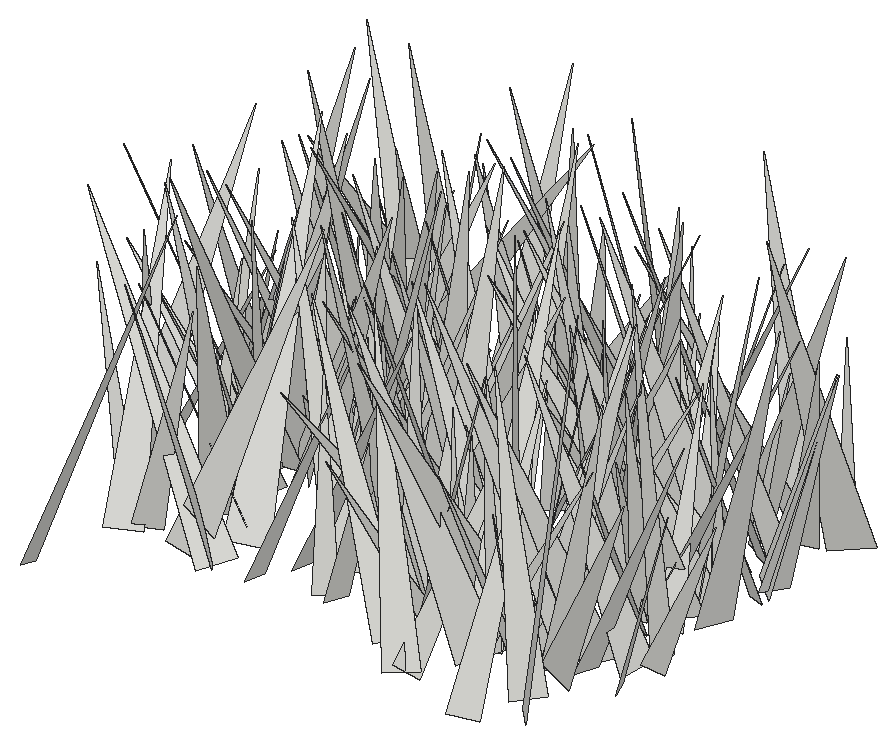
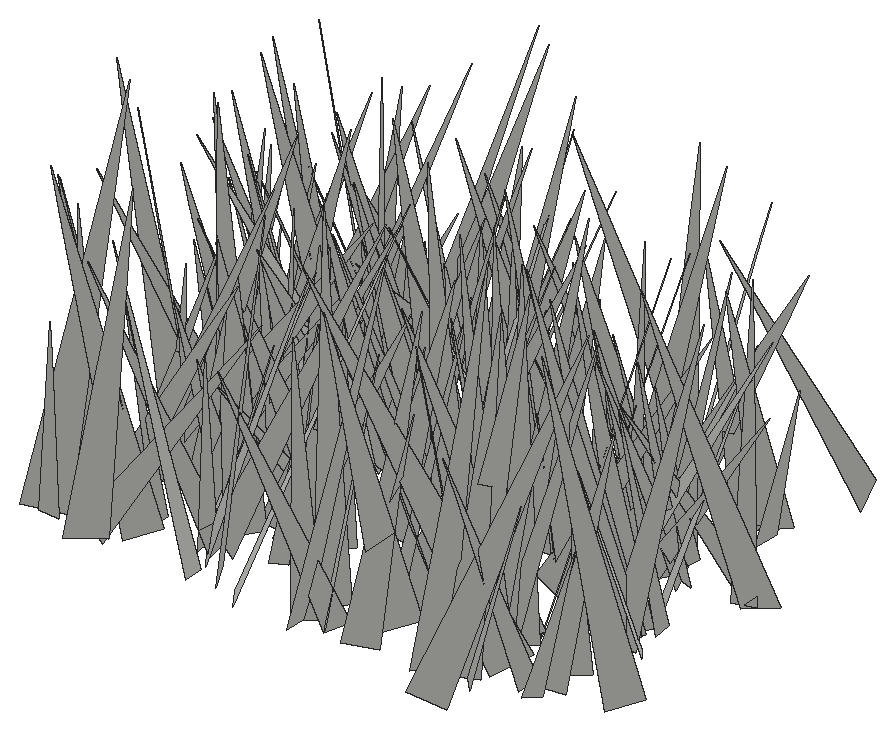
# SketchUp Ruby script. Lengths in inches.
U = 1.inch
M = Sketchup.active_model
def pt(a) = Geom::Point3d.new(a.map { |v| v * U })
def face(e, loops, mat)
  f = e.add_face(loops[0].map { |a| pt(a) })
  loops[1..].each { |l| e.add_face(l.map { |a| pt(a) }).erase! }
  f.material = f.back_material = mat if mat
  f
end
# faces: each face lists its corners as indices into pts; further lists are holes
def faces(e, pts, list, mat = nil) = list.each { |f| face(e, (f[0].is_a?(Array) ? f : [f]).map { |l| l.map { |i| pts[i] } }, mat) }
# xy, xz, yz: faces in a plane at the given z, y or x. An outline is a flat list of corners, or four numbers for a rectangle; further outlines are holes
def ring(l) = l.size == 4 ? [[l[0], l[1]], [l[2], l[1]], [l[2], l[3]], [l[0], l[3]]] : l.each_slice(2).to_a
def flat(e, list, mat, &to3) = list.each { |f| face(e, (f[0].is_a?(Array) ? f : [f]).map { |l| ring(l).map { |u, v| to3.(u, v) } }, mat) }
def xy(e, z, list, mat = nil) = flat(e, list, mat) { |x, y| [x, y, z] }
def xz(e, y, list, mat = nil) = flat(e, list, mat) { |x, z| [x, y, z] }
def yz(e, x, list, mat = nil) = flat(e, list, mat) { |y, z| [x, y, z] }
def lines(e, pts, list) = list.each { |a, b| e.add_line(pt(pts[a]), pt(pts[b])) }
# prism: a flat outline (further loops are holes) pulled along v
def prism(e, loops, v, mat = nil)
  f = face(e, loops, mat); d = Geom::Vector3d.new(v.map { |x| x * U })
  f.pushpull(f.normal.samedirection?(d) ? d.length : -d.length)
end
def box(e, o, s, mat = nil) = prism(e, [[o, [o[0] + s[0], o[1], o[2]], [o[0] + s[0], o[1] + s[1], o[2]], [o[0], o[1] + s[1], o[2]]]], [0, 0, s[2]], mat)
def at(x, y, z, deg = 0) = Geom::Transformation.translation(pt([x, y, z])) * Geom::Transformation.rotation(ORIGIN, Z_AXIS, deg.degrees)
def axes(o, x, y, z) = Geom::Transformation.new([*x, 0, *y, 0, *z, 0, *pt(o).to_a, 1])
def part(name) = M.definitions.add(name)
# library, detail: a bought-in or finely detailed component or shape, given as its bounding box
def library(name, o, s) = part(name).tap { |d| box(d.entities, o, s) }
def detail(e, o, s) = box(e.add_group.entities, o, s)
def put(e, d, t, mat = nil) = e.add_instance(d, t).tap { |i| i.material = mat if mat }
def group(e, t, mat = nil) = e.add_group.tap { |g| g.transformation = t; g.material = mat if mat }.entities
root = M.entities
c1 = part("fur_instance\#9")
p = [[0.8125,0,1.79],[0.67,-0.02,1.48],[0,-0.11,0],[0,0.11,0]]
faces(c1.entities,p,[[0,1,2,3]])
put(root,c1,axes([528.22,20.27,-21.86],[6.68377,2.4417,1.0502],[1.89436,-6.36953,2.75283],[-1.86446,2.28139,6.56175]))
put(root,c1,axes([533.33,24.67,-21.86],[-4.99483,-3.69291,1.05885],[-3.66459,5.10128,0.50484],[1.15306,0.21561,6.19121]))
put(root,c1,axes([545.3125,25.14,-21.86],[-6.87965,3.10007,2.46286],[3.78941,6.58637,2.29475],[1.14737,-3.16466,7.18848]))
put(root,c1,axes([548.58,25.63,-21.86],[0.60809,-6.43634,0.77652],[-5.71222,-0.16309,3.1214],[3.06594,0.97271,5.66154]))
put(root,c1,axes([543.94,22.4375,-21.86],[-2.77056,6.19265,0.76015],[6.19361,2.62958,1.15202],[-0.75223,-1.15721,6.68563]))
put(root,c1,axes([544.375,28.09,-21.86],[-7.59167,-1.95799,2.55179],[-0.44126,7.11339,4.14535],[3.18601,-3.68034,6.65457]))
put(root,c1,axes([548.18,24.13,-21.86],[-2.17091,-2.72609,1.07786],[-2.90812,2.17161,-0.36485],[0.36901,1.07644,3.46573]))
put(root,c1,axes([541.78,26.45,-21.86],[-4.13984,-2.04423,0.54277],[-1.65039,3.86825,1.98107],[1.32277,-1.57147,4.17043]))
put(root,c1,axes([548.81,23.75,-21.86],[-4.49758,4.50366,1.60112],[4.72062,4.53017,0.51777],[0.74986,-1.50644,6.34374]))
put(root,c1,axes([548.17,24.49,-21.86],[-1.77005,-3.87903,0.89181],[-3.77258,1.32393,-1.7292],[-1.26879,1.475,3.89741]))
put(root,c1,axes([549.52,22.64,-21.86],[5.31201,5.41879,2.20999],[5.24419,-5.73235,1.45032],[-2.59727,-0.49162,7.44831]))
put(root,c1,axes([530,25.04,-21.86],[3.51302,-4.23345,1.0034],[-4.35037,-3.40123,0.88101],[0.05668,1.33409,5.43021]))
put(root,c1,axes([547.81,21.18,-21.86],[-5.23053,3.77379,0.03544],[3.44734,4.80229,-2.57973],[1.53577,2.07308,5.91142]))
put(root,c1,axes([542.18,24.05,-21.86],[-3.49983,5.63032,0.78088],[5.54982,3.18646,1.89866],[-1.22869,-1.64469,6.35172]))
put(root,c1,axes([531.5,27.51,-21.86],[4.72004,-5.82808,0.22381],[-5.80637,-4.72269,-0.52693],[-0.55017,-0.15829,7.48115]))
put(root,c1,axes([532.24,24.45,-21.86],[-0.29437,7.39176,2.68978],[7.28817,1.26884,-2.68928],[2.95898,-2.3899,6.89148]))
put(root,c1,axes([533.66,24.48,-21.86],[-4.54084,5.90887,0.08971],[5.53212,4.21055,2.68494],[-2.07809,-1.7025,6.95162]))
put(root,c1,axes([542.27,25.55,-21.86],[5.73054,2.09287,1.0832],[2.24178,-5.71944,-0.8093],[-0.7265,-1.14039,6.04684]))
put(root,c1,axes([538.19,25.17,-21.86],[-2.40866,3.6867,1.3913],[3.88066,2.50239,0.08743],[0.68406,-1.21467,4.40293]))
put(root,c1,axes([535.37,24.59,-21.86],[5.62442,0.34622,0.61815],[0.22701,-5.5658,1.05184],[-0.67115,1.01884,5.53603]))
put(root,c1,axes([545.3,25.47,-21.86],[3.75203,3.55416,0.24846],[3.4305,-3.50645,-1.64561],[0.96201,-1.35805,4.89916]))
put(root,c1,axes([549.14,27.58,-21.86],[2.35436,-6.19743,2.05043],[-5.78585,-2.99044,-2.39512],[-3.02263,0.89697,6.18179]))
put(root,c1,axes([539.05,29.83,-21.86],[-5.34969,-3.46152,0.37635],[-2.75195,4.62606,3.43064],[2.1332,-2.713,5.36954]))
put(root,c1,axes([548.21,26.17,-21.86],[5.31281,-2.73186,1.51927],[-2.91837,-5.40827,0.48055],[-1.11999,1.13346,5.95467]))
put(root,c1,axes([548.04,27.38,-21.86],[-8.03194,-0.35365,0.82088],[-0.22203,7.97883,1.26494],[0.86581,-1.23463,7.93959]))
put(root,c1,axes([540.31,27.43,-21.86],[-1.48143,-7.59825,2.03928],[-7.84224,1.26126,-0.99758],[-0.62555,2.18232,7.67677]))
put(root,c1,axes([536.26,26.47,-21.86],[6.32443,-0.86949,0.03215],[-0.87008,-6.31952,0.24926],[0.00213,0.25131,6.37905]))
put(root,c1,axes([529.03,25.28,-21.86],[-4.67353,1.04438,0.03845],[1.02272,4.60667,-0.8165],[0.21505,0.78861,4.71868]))
put(root,c1,axes([545.79,25.68,-21.86],[-4.82421,0.67017,1.12309],[0.52178,4.9221,-0.69578],[1.19925,0.5543,4.82058]))
put(root,c1,axes([544.24,25.28,-21.86],[0.68638,4.30492,0.85677],[4.11958,-0.93113,1.37825],[-1.51508,-0.58153,4.13569]))
put(root,c1,axes([544.08,22.53,-21.86],[-5.06896,3.36354,0.19703],[2.56301,4.08037,-3.71862],[2.18706,3.01393,4.81452]))
put(root,c1,axes([550.95,26.39,-21.86],[3.66327,1.41122,0.72087],[1.44956,-3.71776,-0.08822],[-0.64027,-0.34277,3.92471]))
put(root,c1,axes([529.375,24.4,-21.86],[-3.85678,5.81728,0.33644],[5.7739,3.8696,-0.71896],[0.78484,0.11882,6.94252]))
put(root,c1,axes([550.54,27.97,-21.86],[-6.51837,1.52305,1.37348],[1.82295,6.39951,1.5551],[0.93967,-1.84981,6.5108]))
put(root,c1,axes([547.09,25.1875,-21.86],[-7.31055,-2.64435,2.80127],[-3.45475,7.15889,-2.25809],[1.70424,3.16886,7.43894]))
put(root,c1,axes([532.53,27.58,-21.86],[-3.6362,-3.51378,0.23491],[-3.4583,3.49912,-1.19165],[-0.6648,1.01649,4.91412]))
put(root,c1,axes([549.14,26.72,-21.86],[5.55155,-0.72144,0.45458],[-0.77671,-5.51397,0.73462],[-0.35191,0.78896,5.54982]))
put(root,c1,axes([545.98,26.65,-21.86],[-4.87029,1.64927,0.93909],[1.65484,4.95663,-0.12272],[0.92923,-0.18296,5.1405]))
put(root,c1,axes([542.8,27.73,-21.86],[2.98723,-2.64764,1.00912],[-2.72025,-3.09017,-0.05514],[-0.79284,0.62671,3.99131]))
put(root,c1,axes([542.49,28.64,-21.86],[-3.80657,-5.75041,0.9295],[-5.82495,3.76407,-0.56819],[0.03325,1.08891,6.87272]))
put(root,c1,axes([546.9,27.07,-21.86],[3.44666,-5.98968,2.82803],[-6.61551,-2.95389,1.80641],[0.33028,3.33943,6.67028]))
put(root,c1,axes([538.6875,25.21,-21.86],[-7.17026,0.40545,3.85637],[-0.86926,7.73252,-2.42922],[3.77894,2.54801,6.75839]))
put(root,c1,axes([539.45,29.11,-21.86],[4.28198,-1.79299,1.3249],[-1.43721,-4.41332,-1.32759],[-1.70429,-0.78312,4.44833]))
put(root,c1,axes([551.01,28.27,-21.86],[2.19638,-3.75423,0.49776],[-3.62923,-1.92217,1.51658],[1.08198,1.1735,4.07656]))
put(root,c1,axes([539.53,27.79,-21.86],[-3.51582,-2.14374,0.80605],[-2.26912,3.46073,-0.69338],[0.31056,1.01688,4.05904]))
put(root,c1,axes([537.68,26.9,-21.86],[-2.86561,6.0597,1.12131],[6.09085,2.59686,1.53195],[-0.93747,-1.65086,6.5257]))
put(root,c1,axes([526.68,29.48,-21.86],[-0.27546,-6.0552,1.07535],[-6.00995,0.49341,1.23885],[1.30474,0.99438,5.93351]))
put(root,c1,axes([546.91,26.4375,-21.86],[3.10305,4.72146,0.30771],[4.72969,-3.10544,-0.04628],[-0.13026,-0.28259,5.64969]))
put(root,c1,axes([538.18,28.74,-21.86],[-0.76363,-5.08076,1.72351],[-5.30047,0.98391,0.55201],[0.83046,1.60796,5.10809]))
put(root,c1,axes([540.88,26.92,-21.86],[-5.6137,1.8249,1.28834],[1.63706,5.7317,-0.98561],[1.51991,0.56669,5.82001]))
put(root,c1,axes([545.02,25.62,-21.86],[-2.31741,7.72302,0.72504],[7.71845,2.37113,-0.58682],[0.77216,-0.52327,8.04183]))
put(root,c1,axes([548.56,30.52,-21.86],[-1.70648,-4.83175,0.15849],[-4.67215,1.69151,1.26205],[1.24174,-0.27565,4.96639]))
put(root,c1,axes([531.08,31.69,-21.86],[0.62863,-8.27068,0.12443],[-8.26435,-0.63324,-0.33804],[-0.34653,0.09834,8.28764]))
put(root,c1,axes([531.95,30.14,-21.86],[2.79879,-2.29313,0.37979],[-2.08936,-2.74248,-1.16161],[-1.01846,-0.6755,3.42672]))
put(root,c1,axes([535.9375,27.78,-21.86],[3.61402,1.40651,0.81578],[1.29809,-3.69316,0.61679],[-0.97915,0.29527,3.8287]))
put(root,c1,axes([537.5,33.42,-21.86],[-5.2335,-6.40482,0.23356],[-5.52847,4.66397,4.0186],[3.24225,-2.38569,7.22925]))
put(root,c1,axes([530.58,29.44,-21.86],[-6.31827,-0.38458,1.65434],[-0.20418,6.49842,0.73085],[1.68614,-0.65417,6.28763]))
put(root,c1,axes([531.88,27.46,-21.86],[4.20978,2.5999,1.29958],[2.36123,-4.39284,1.13935],[-1.69498,0.33775,4.81493]))
put(root,c1,axes([530.62,30.41,-21.86],[-1.9531,-3.93926,0.49775],[-3.87343,2.01224,0.72636],[0.87298,0.11511,4.33645]))
put(root,c1,axes([536.91,29.01,-21.86],[-0.32853,3.96848,1.56907],[4.26678,0.33258,0.05223],[0.07349,-1.56822,3.98171]))
put(root,c1,axes([543.24,29.33,-21.86],[-5.49496,2.98551,0.84144],[3.09795,5.36781,1.18541],[0.15494,-1.44541,6.14025]))
put(root,c1,axes([530.94,30.68,-21.86],[-1.97091,-5.99186,1.73382],[-5.97714,2.33419,1.27215],[1.7839,1.20092,6.17807]))
put(root,c1,axes([533.61,26.28,-21.86],[-2.88963,7.72101,0.14725],[7.7077,2.8933,-0.45358],[0.4764,0.02131,8.23153]))
put(root,c1,axes([541.88,30.5625,-21.86],[0.38747,-3.62863,0.53891],[-3.66751,-0.39531,-0.02484],[-0.08219,0.53319,3.64917]))
put(root,c1,axes([530.11,28.46,-21.86],[3.76541,-0.98312,2.37268],[-1.72485,-4.08783,1.04352],[-1.9029,1.75998,3.74912]))
put(root,c1,axes([544.96,27.7,-21.86],[-5.36407,2.31527,0.60969],[2.0889,5.25672,-1.5839],[1.1699,1.22955,5.6236]))
put(root,c1,axes([548.52,30.96,-21.86],[5.03393,-2.19184,1.50174],[-1.99616,-5.24318,-0.96135],[-1.75349,-0.32355,5.40559]))
put(root,c1,axes([533.46,28.37,-21.86],[3.44436,3.22324,0.28553],[3.18394,-3.45028,0.54084],[-0.57733,0.20181,4.68619]))
put(root,c1,axes([545.22,28.35,-21.86],[3.77893,2.89431,1.05154],[2.64296,-3.90266,1.24382],[-1.58036,0.3941,4.59459]))
put(root,c1,axes([539.42,30.3,-21.86],[1.67696,-6.87357,2.26471],[-6.67493,-0.57073,3.21041],[2.79647,2.7596,6.30488]))
put(root,c1,axes([540.58,31.24,-21.86],[-6.39849,-1.36399,1.46981],[-1.16574,6.52941,0.98452],[1.63152,-0.68393,6.46776]))
put(root,c1,axes([528.54,32.22,-21.86],[-3.05725,-3.63504,0.09512],[-3.51202,2.98398,1.15363],[0.94245,-0.67208,4.60753]))
put(root,c1,axes([530.66,30.58,-21.86],[-4.24155,2.82864,0.08548],[2.61337,3.85608,2.07369],[-1.08573,-1.76881,4.65744]))
put(root,c1,axes([547.71,31.64,-21.86],[4.05773,-0.76512,0.97615],[-0.40955,-3.97873,-1.41614],[-1.1707,-1.26007,3.87881]))
put(root,c1,axes([550.81,29.1,-21.86],[-7.01031,-0.43579,1.43561],[-0.72042,6.99511,-1.39453],[1.31601,1.50792,6.88401]))
put(root,c1,axes([540.61,28.99,-21.86],[-4.94866,6.16749,2.69055],[6.18584,5.48419,-1.19385],[2.6481,-1.28527,7.81677]))
put(root,c1,axes([527.6,28.3,-21.86],[4.79921,1.03907,0.41248],[0.79797,-4.45725,1.94381],[-0.78297,1.82633,4.50929]))
put(root,c1,axes([530.29,29.76,-21.86],[-2.58112,4.19595,2.18678],[4.13957,3.20902,-1.27135],[2.29171,-1.07069,4.75939]))
put(root,c1,axes([531.29,30.875,-21.86],[-5.24888,-4.54366,0.15791],[-4.36596,4.97023,-2.11085],[-1.26815,1.69482,6.61361]))
put(root,c1,axes([539.43,30.16,-21.86],[-6.20853,-2.44848,0.56631],[-2.51301,6.03462,-1.45936],[-0.02325,1.56521,6.51238]))
put(root,c1,axes([549.61,32.21,-21.86],[1.87791,-4.76016,0.94457],[-4.63856,-2.05833,-1.15104],[-1.42657,0.4266,4.98606]))
put(root,c1,axes([531.2,32.21,-21.86],[4.92449,-2.5321,0.51516],[-2.43841,-4.92066,-0.87679],[-0.85503,-0.55051,5.46748]))
put(root,c1,axes([533.17,32.86,-21.86],[-0.84326,-5.89202,0.02664],[-5.53518,0.78295,-2.04363],[-2.01949,0.3143,5.59022]))
put(root,c1,axes([537.55,28.43,-21.86],[4.61833,5.37447,0.17353],[5.34108,-4.61135,0.67253],[-0.62281,0.30742,7.05419]))
put(root,c1,axes([526.06,29.27,-21.86],[-1.22058,7.14872,1.6543],[7.02907,1.62036,-1.81584],[2.10547,-1.26529,7.02116]))
put(root,c1,axes([531.89,32.44,-21.86],[2.97269,-7.01093,0.81561],[-6.80259,-2.60982,2.35986],[1.88234,1.64042,7.24024]))
put(root,c1,axes([529.64,29.4,-21.86],[5.0446,1.96996,1.21492],[1.59207,-5.06819,1.60732],[-1.6799,1.1124,5.17158]))
put(root,c1,axes([548.07,30.56,-21.86],[-0.49595,7.7495,2.67586],[7.77568,-0.40515,2.61451],[-2.59882,-2.6911,7.31198]))
put(root,c1,axes([529.72,29.46,-21.86],[0.92539,5.82013,0.73982],[5.78512,-1.02986,0.86568],[-0.97656,-0.58571,5.82931]))
put(root,c1,axes([546.22,27.79,-21.86],[-5.33853,3.8285,0.2094],[3.37353,4.86067,-2.86257],[1.82225,2.21756,5.91295]))
put(root,c1,axes([532.26,31.6,-21.86],[3.37975,2.64749,1.02841],[2.82915,-3.2791,-0.85611],[-0.25046,-1.31446,4.20701]))
put(root,c1,axes([541.5625,31.34,-21.86],[-2.08975,2.94897,0.92989],[3.09202,1.98432,0.65582],[-0.0238,-1.13764,3.55435]))
put(root,c1,axes([528.45,33.42,-21.86],[0.97454,-6.53217,0.4424],[-5.83998,-0.6651,3.04417],[2.95966,0.83851,5.86106]))
put(root,c1,axes([544.7,31.74,-21.86],[7.35605,-1.97253,1.00478],[-2.03855,-7.39535,0.40615],[-0.86301,0.65556,7.60509]))
put(root,c1,axes([531.28,34.37,-21.86],[-5.93761,-4.29126,0.84113],[-3.95201,5.87307,2.0655],[1.8719,-1.21235,7.02879]))
put(root,c1,axes([538.6,31.94,-21.86],[5.35038,-4.23141,0.69897],[-4.27634,-5.17862,1.38378],[0.32603,1.51562,6.67957]))
put(root,c1,axes([534.96,30.99,-21.86],[-0.41482,4.98169,1.32883],[5.15587,0.40286,0.09923],[0.00793,-1.33251,4.99795]))
put(root,c1,axes([543.75,29.11,-21.86],[7.40987,3.38689,0.1989],[3.26816,-7.25381,1.76579],[-0.91088,1.52574,7.95356]))
put(root,c1,axes([550.63,32.31,-21.86],[6.87118,-2.4682,1.14103],[-2.53265,-6.93781,0.24398],[-0.98977,0.61792,7.29696]))
put(root,c1,axes([543.64,32.25,-21.86],[5.88028,2.97965,0.94292],[3.11911,-5.72141,-1.37172],[-0.19635,-1.65292,6.44782]))
put(root,c1,axes([544.87,31.78,-21.86],[3.6305,3.98779,0.322],[3.84064,-3.3521,-1.78874],[1.12055,-1.43096,5.08758]))
put(root,c1,axes([549.64,30.92,-21.86],[-2.09366,4.25191,0.8072],[4.26644,2.17826,-0.40798],[0.72654,-0.53866,4.72184]))
put(root,c1,axes([544.6,34.23,-21.86],[6.00758,0.21792,0.49644],[0.387,-5.59183,-2.22857],[-0.3797,-2.2514,5.58318]))
put(root,c1,axes([530.99,35.91,-21.86],[-5.78164,-4.6449,0.78576],[-4.06196,5.54542,2.89287],[2.386,-1.8147,6.82889]))
put(root,c1,axes([545.25,33.22,-21.86],[-2.5079,-4.6968,1.95628],[-4.90602,2.8103,0.45782],[1.34828,1.48955,5.3047]))
put(root,c1,axes([543.55,34.55,-21.86],[5.83634,-0.86723,1.56304],[-0.35494,-5.79341,-1.88904],[-1.75191,-1.71533,5.58985]))
put(root,c1,axes([546.17,34.64,-21.86],[-6.77007,0.71674,0.61078],[0.8862,6.3486,2.37288],[0.31848,-2.42944,6.38099]))
put(root,c1,axes([536.82,33.67,-21.86],[2.7668,-7.06079,2.0724],[-7.35623,-2.5972,0.97226],[0.18857,2.28135,7.52095]))
put(root,c1,axes([528.35,34.58,-21.86],[-0.27695,-6.43694,1.01641],[-6.49492,0.18954,-0.56932],[-0.53231,1.03627,6.4177]))
put(root,c1,axes([548.53,33.34,-21.86],[-2.71557,-5.16024,0.69315],[-4.67023,2.06855,-2.89705],[-2.30163,1.89099,5.06058]))
put(root,c1,axes([527.8,32.86,-21.86],[4.33952,0.70183,1.00017],[0.70812,-4.45199,0.05164],[-0.99573,-0.10739,4.3956]))
put(root,c1,axes([548.58,31.38,-21.86],[6.37696,0.70596,0.43543],[0.57496,-6.19552,1.62437],[-0.59783,1.57187,6.20688]))
put(root,c1,axes([542.61,30.01,-21.86],[0.71123,8.26754,0.30404],[8.18462,-0.74766,1.1847],[-1.20692,-0.19821,8.21307]))
put(root,c1,axes([549.63,33.18,-21.86],[-2.51256,7.06983,2.10699],[6.38069,0.96553,4.36915],[-3.70253,-3.13371,6.09968]))
put(root,c1,axes([536.22,32.11,-21.86],[2.59525,5.12132,1.23508],[5.09738,-2.78884,0.85303],[-1.33041,-0.69505,5.67763]))
put(root,c1,axes([533.76,31.74,-21.86],[2.74983,3.97442,1.3241],[3.39736,-3.04242,2.07665],[-2.45097,0.24187,4.36407]))
put(root,c1,axes([537.07,34.125,-21.86],[-6.53044,0.59698,0.86107],[0.69842,6.53195,0.76827],[0.78105,-0.84949,6.51251]))
put(root,c1,axes([543.33,33.09,-21.86],[5.01849,-2.22986,0.6447],[-2.32023,-4.77497,1.54574],[0.06662,1.67347,5.26955]))
put(root,c1,axes([537.73,32.56,-21.86],[2.61038,6.20008,1.07332],[6.21386,-2.35716,-1.49626],[0.99041,-1.55238,6.55868]))
put(root,c1,axes([543.84,35.68,-21.86],[1.73038,-3.85975,0.19684],[-3.59553,-1.68683,-1.46882],[-1.41726,-0.43309,3.96667]))
put(root,c1,axes([548.72,33.58,-21.86],[-3.91032,-4.73518,3.93684],[-5.20514,5.03349,0.88414],[3.29046,2.33522,6.07707]))
put(root,c1,axes([550.42,33.02,-21.86],[0.93593,4.40998,1.37185],[4.37962,-1.29175,1.16453],[-1.46587,-1.0437,4.3552]))
put(root,c1,axes([550.6875,34.6875,-21.86],[-2.25031,-4.2676,0.76277],[-4.32128,2.13921,-0.77999],[-0.34742,1.03417,4.76108]))
put(root,c1,axes([533.04,35.26,-21.86],[-1.51779,-7.89387,2.17922],[-8.18213,1.37007,-0.73587],[-0.33897,2.275,8.00471]))
put(root,c1,axes([548.8,35.48,-21.86],[2.25381,-7.00366,2.80187],[-6.80723,-3.14832,-2.39397],[-3.25014,1.7373,6.957]))
put(root,c1,axes([528.47,34.15,-21.86],[4.89354,-4.52263,1.72188],[-4.82903,-4.72322,1.31813],[-0.31551,2.14541,6.53173]))
put(root,c1,axes([536.45,37.18,-21.86],[-1.51333,-7.7582,0.0595],[-7.60064,1.47034,-1.59746],[-1.5568,0.36304,7.74132]))
put(root,c1,axes([540.14,33.45,-21.86],[-2.07893,6.71015,1.41675],[6.64432,1.60395,2.15305],[-1.69892,-1.93817,6.68674]))
put(root,c1,axes([531.94,36.74,-21.86],[6.8807,-3.2851,0.24825],[-3.20439,-6.80705,-1.26238],[-0.76512,-1.03432,7.51946]))
put(root,c1,axes([540.74,35.32,-21.86],[2.93376,-3.22318,1.07266],[-3.3076,-3.03341,-0.06853],[-0.77414,0.74566,4.35788]))
put(root,c1,axes([545.19,35.75,-21.86],[4.39252,-6.51911,2.0007],[-6.79057,-4.39945,0.57342],[-0.62428,1.98542,7.83991]))
put(root,c1,axes([528.1,34.42,-21.86],[7.69259,-0.4984,1.40276],[-0.64413,-7.77059,0.77146],[-1.3421,0.87272,7.67002]))
put(root,c1,axes([527.3125,34.65,-21.86],[2.99336,2.37967,0.42143],[2.41657,-2.95437,-0.48225],[-0.02533,-0.63994,3.79348]))
put(root,c1,axes([544.18,36.73,-21.86],[7.73764,-3.02475,0.93063],[-2.93122,-7.77665,-0.90436],[-1.19293,-0.51074,8.25847]))
put(root,c1,axes([531.24,36.94,-21.86],[5.34448,-4.72432,0.68412],[-4.69665,-5.3877,-0.51471],[-0.85369,0.0645,7.11462]))
put(root,c1,axes([550.375,35.57,-21.86],[3.55889,4.26793,1.49162],[4.48448,-3.09137,-1.85436],[0.57409,-2.30955,5.23854]))
put(root,c1,axes([550.77,35.69,-21.86],[5.12871,-2.48578,0.55768],[-2.53054,-5.11559,0.47007],[-0.29413,0.66743,5.67995]))
put(root,c1,axes([544.31,32.77,-21.86],[3.66299,2.22216,0.32756],[1.7102,-3.16536,2.34915],[-1.4562,1.87225,3.58288]))
put(root,c1,axes([536.77,37.27,-21.86],[-3.08937,-5.14938,0.76665],[-5.09175,3.1744,0.80332],[1.08532,0.23487,5.95105]))
put(root,c1,axes([531.37,37.95,-21.86],[-0.1774,-7.7519,1.13116],[-7.17611,0.61466,3.08685],[3.14245,0.96602,7.113]))
put(root,c1,axes([531.82,36.89,-21.86],[-2.67742,-5.68655,1.10676],[-5.79247,2.6077,-0.61446],[-0.09527,1.2623,6.25523]))
put(root,c1,axes([542.49,36.23,-21.86],[-4.33976,4.07233,1.17149],[4.17045,3.80756,2.21352],[-0.75076,-2.38923,5.52429]))
put(root,c1,axes([541.85,37.69,-21.86],[4.21418,-1.38432,0.79636],[-0.98829,-4.02576,-1.76817],[-1.25452,-1.47878,4.06808]))
put(root,c1,axes([548.42,34.05,-21.86],[-4.08982,2.78235,0.32679],[2.66533,4.04258,-1.06229],[0.86271,0.7007,4.83111]))
put(root,c1,axes([542.14,35.77,-21.86],[-2.43911,-2.15453,1.73505],[-2.51562,2.68975,-0.19638],[1.15067,1.31336,3.24849]))
put(root,c1,axes([543.39,34.65,-21.86],[-1.53438,4.71255,0.03454],[4.47921,1.44703,1.55125],[-1.46492,-0.51147,4.70702]))
put(root,c1,axes([549.09,37.08,-21.86],[-4.74845,-6.02691,1.04144],[-6.05438,4.44477,-1.88271],[-0.8676,1.96887,7.4382]))
put(root,c1,axes([540.66,37.4,-21.86],[0.4786,-6.17329,1.68247],[-6.39725,-0.42884,0.2463],[0.12453,1.69584,6.18692]))
put(root,c1,axes([544.44,37.74,-21.86],[-3.30387,-7.05223,0.96215],[-6.92829,2.9435,-2.21582],[-1.63048,1.78244,7.4659]))
put(root,c1,axes([531.41,36.22,-21.86],[3.36914,-5.54095,2.01408],[-5.73384,-2.5398,2.60427],[1.37175,2.99283,5.93894]))
put(root,c1,axes([535.2,36.52,-21.86],[2.4928,2.63766,0.46244],[2.65596,-2.35455,-0.88721],[0.34203,-0.94022,3.51911]))
put(root,c1,axes([547.26,35.55,-21.86],[-1.00856,5.27208,0.80529],[5.17147,0.76643,1.45913],[-1.30357,-1.0384,5.16556]))
put(root,c1,axes([546.37,34.74,-21.86],[-4.2837,1.86088,0.37109],[1.60299,4.03921,-1.75094],[1.01537,1.47394,4.32979]))
put(root,c1,axes([544.8,37.85,-21.86],[-3.61548,-1.81279,0.7212],[-1.71327,3.67656,0.65243],[0.9333,-0.2734,3.99152]))
put(root,c1,axes([532.08,37.49,-21.86],[0.54062,-3.9189,1.26852],[-4.01221,-0.79056,-0.73238],[-0.93225,1.12979,3.88763]))
put(root,c1,axes([545.55,35.71,-21.86],[-2.74828,4.07366,1.32335],[3.94461,3.01992,-1.10419],[1.66916,-0.42944,4.78838]))
put(root,c1,axes([545.42,37.34,-21.86],[-5.70122,-3.26457,0.62497],[-3.32356,5.6155,-0.98593],[0.04408,1.16649,6.49533]))
put(root,c1,axes([551.06,39.83,-21.86],[4.03591,-7.21522,0.98619],[-7.10178,-4.1491,-1.2924],[-1.61145,0.21471,8.16564]))
put(root,c1,axes([549.47,38.93,-21.86],[2.80299,-5.03768,0.10257],[-5.00094,-2.76705,0.76127],[0.6159,0.45904,5.71449]))
put(root,c1,axes([528.05,37.28,-21.86],[-2.23187,2.81976,1.51549],[3.01775,2.4697,-0.15093],[1.06816,-1.08561,3.59298]))
put(root,c1,axes([533.66,37.06,-21.86],[-4.16616,6.68617,2.08588],[7.00105,3.90518,1.46546],[-0.20279,-2.54114,7.74043]))
put(root,c1,axes([541.5,40.74,-21.86],[-6.65977,-5.09555,0.25994],[-4.96209,6.56797,1.61994],[1.1874,-1.13219,8.22757]))
put(root,c1,axes([528.22,38.82,-21.86],[1.56838,-4.91392,1.31708],[-4.91027,-1.82266,-0.95305],[-1.33063,0.93404,5.06933]))
put(root,c1,axes([547.2,37.91,-21.86],[4.1341,0.32333,0.78637],[0.3951,-4.18703,-0.35553],[-0.75288,-0.42186,4.13146]))
put(root,c1,axes([531.38,40.15,-21.86],[3.47226,-5.91321,0.27335],[-5.89868,-3.48291,-0.41506],[-0.49636,0.02495,6.84473]))
put(root,c1,axes([549.73,37.41,-21.86],[-2.26256,-5.81888,2.33683],[-5.71547,0.89178,-3.31322],[-2.57945,3.12805,5.2916]))
put(root,c1,axes([538.26,39.05,-21.86],[7.26083,-2.43104,1.92439],[-2.31077,-7.51014,-0.76873],[-2.06726,-0.14373,7.61831]))
put(root,c1,axes([533.03,37.62,-21.86],[-3.67972,-3.6806,3.42599],[-4.33109,4.47676,0.15761],[2.55458,2.28831,5.20214]))
put(root,c1,axes([548.22,37.64,-21.86],[1.71748,3.11444,0.84575],[3.20742,-1.75327,-0.057],[-0.35706,-0.7688,3.55615]))
put(root,c1,axes([525.4,38.03,-21.86],[5.70203,-3.94241,1.833],[-4.2894,-5.59456,1.31056],[-0.70959,2.13867,6.80721]))
put(root,c1,axes([531.29,42.29,-21.86],[4.10096,-6.21113,0.1393],[-5.64172,-3.79303,-3.03306],[-2.60165,-1.56533,6.79681]))
put(root,c1,axes([530.48,38.28,-21.86],[5.80573,-6.03364,0.3689],[-5.4436,-4.99608,3.95649],[2.62833,2.98023,7.37953]))
put(root,c1,axes([537.6,40.35,-21.86],[-3.59225,-3.71334,1.0598],[-3.39845,3.72735,1.54069],[1.83374,-0.36648,4.93148]))
put(root,c1,axes([537.82,37.17,-21.86],[-5.65883,0.17912,0.29432],[0.09895,5.4838,-1.43499],[0.33003,1.4272,5.47679]))
put(root,c1,axes([547.05,39.09,-21.86],[6.03076,-3.95506,0.64167],[-4.00583,-5.92637,1.12057],[0.08689,1.28836,7.12438]))
put(root,c1,axes([532.68,40.28,-21.86],[6.98287,-2.99298,2.96369],[-2.61118,-7.57832,-1.50091],[-3.30502,-0.33623,7.44753]))
put(root,c1,axes([535.7,40.6,-21.86],[3.60817,-5.34608,1.25489],[-5.24687,-3.79935,-1.09972],[-1.62036,0.39817,6.35531]))
put(root,c1,axes([544.51,38.57,-21.86],[-6.0406,-4.0795,1.11122],[-4.22494,5.74856,-1.86274],[-0.16426,2.16279,7.04708]))
put(root,c1,axes([548.75,39.91,-21.86],[-1.84266,-5.86998,0.99209],[-5.21002,1.08759,-3.24178],[-2.88039,1.78795,5.22904]))
put(root,c1,axes([544.33,38.04,-21.86],[6.26365,0.83218,0.34032],[0.77044,-6.2027,0.98722],[-0.46342,0.93576,6.24109]))
put(root,c1,axes([544.83,38.12,-21.86],[-4.924,0.48292,1.1816],[0.20052,4.94285,-1.18453],[1.26062,1.10005,4.80373]))
put(root,c1,axes([542.94,39.79,-21.86],[-6.29622,-3.82649,2.40942],[-4.00808,6.63484,0.06324],[2.09347,1.19444,7.36752]))
put(root,c1,axes([529.11,39.02,-21.86],[4.6922,-0.3007,0.23761],[-0.32477,-4.66947,0.50417],[-0.20347,0.51889,4.67471]))
put(root,c1,axes([538.55,40.67,-21.86],[-7.391,-1.41623,2.02124],[-1.14457,7.62073,1.15434],[2.18657,-0.79801,7.4364]))
put(root,c1,axes([538.45,40.26,-21.86],[2.86346,-4.49186,1.0378],[-4.60706,-2.8331,0.44926],[-0.16992,1.11803,5.30796]))
put(root,c1,axes([543.78,40.26,-21.86],[6.21728,1.67139,0.47713],[1.73743,-6.02723,-1.52629],[-0.05031,-1.59834,6.25448]))
put(root,c1,axes([528.4375,39.63,-21.86],[-3.21224,1.96871,0.46482],[2.01704,3.18335,0.45637],[0.15311,-0.63315,3.7398]))
put(root,c1,axes([530.83,40.35,-21.86],[-2.84095,-2.72325,0.75235],[-2.80656,2.8428,-0.30791],[0.32453,0.74533,3.9233]))
put(root,c1,axes([537.21,40.05,-21.86],[2.54302,-4.52945,1.06711],[-4.23804,-1.75205,2.66287],[1.92189,2.12978,4.46004]))
put(root,c1,axes([550.7,40.04,-21.86],[-0.06677,3.94377,1.582],[4.24655,0.00562,0.16522],[-0.15123,-1.5834,3.94087]))
put(root,c1,axes([535.44,38.5625,-21.86],[5.43285,-3.6045,3.64876],[-4.74936,-5.54221,1.59663],[-1.93634,3.48041,6.32132]))
put(root,c1,axes([548.55,40.57,-21.86],[-5.45216,4.70878,2.71596],[5.23215,5.58914,0.81316],[1.47433,-2.42158,7.15803]))
